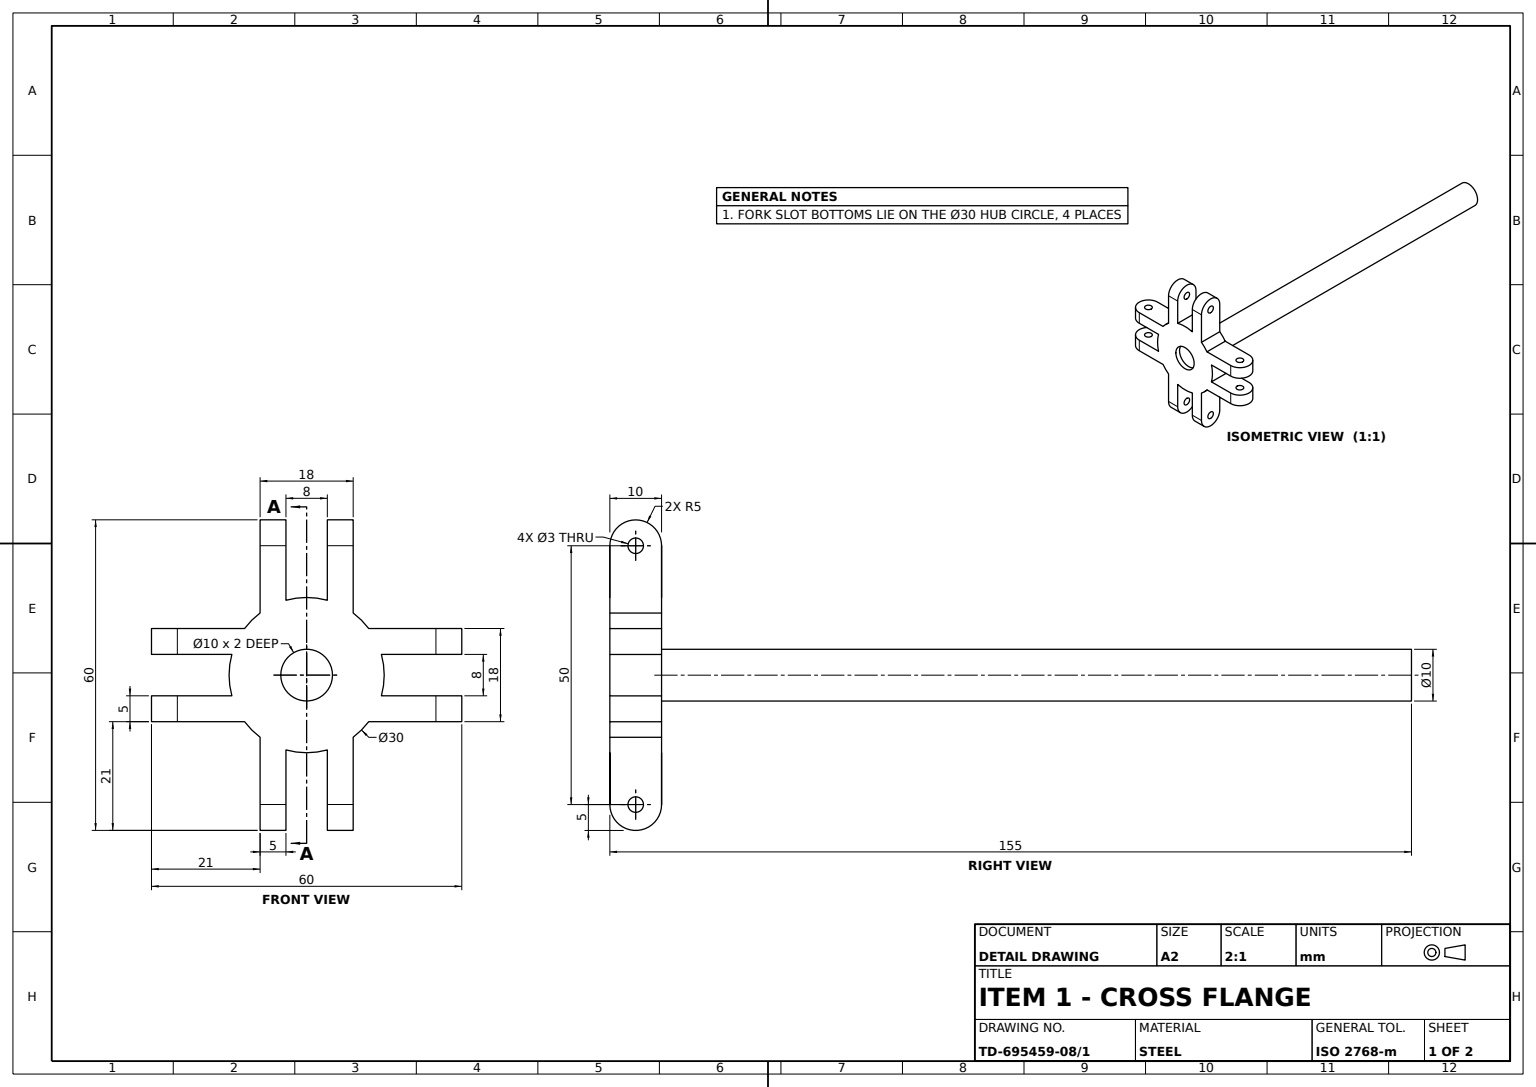
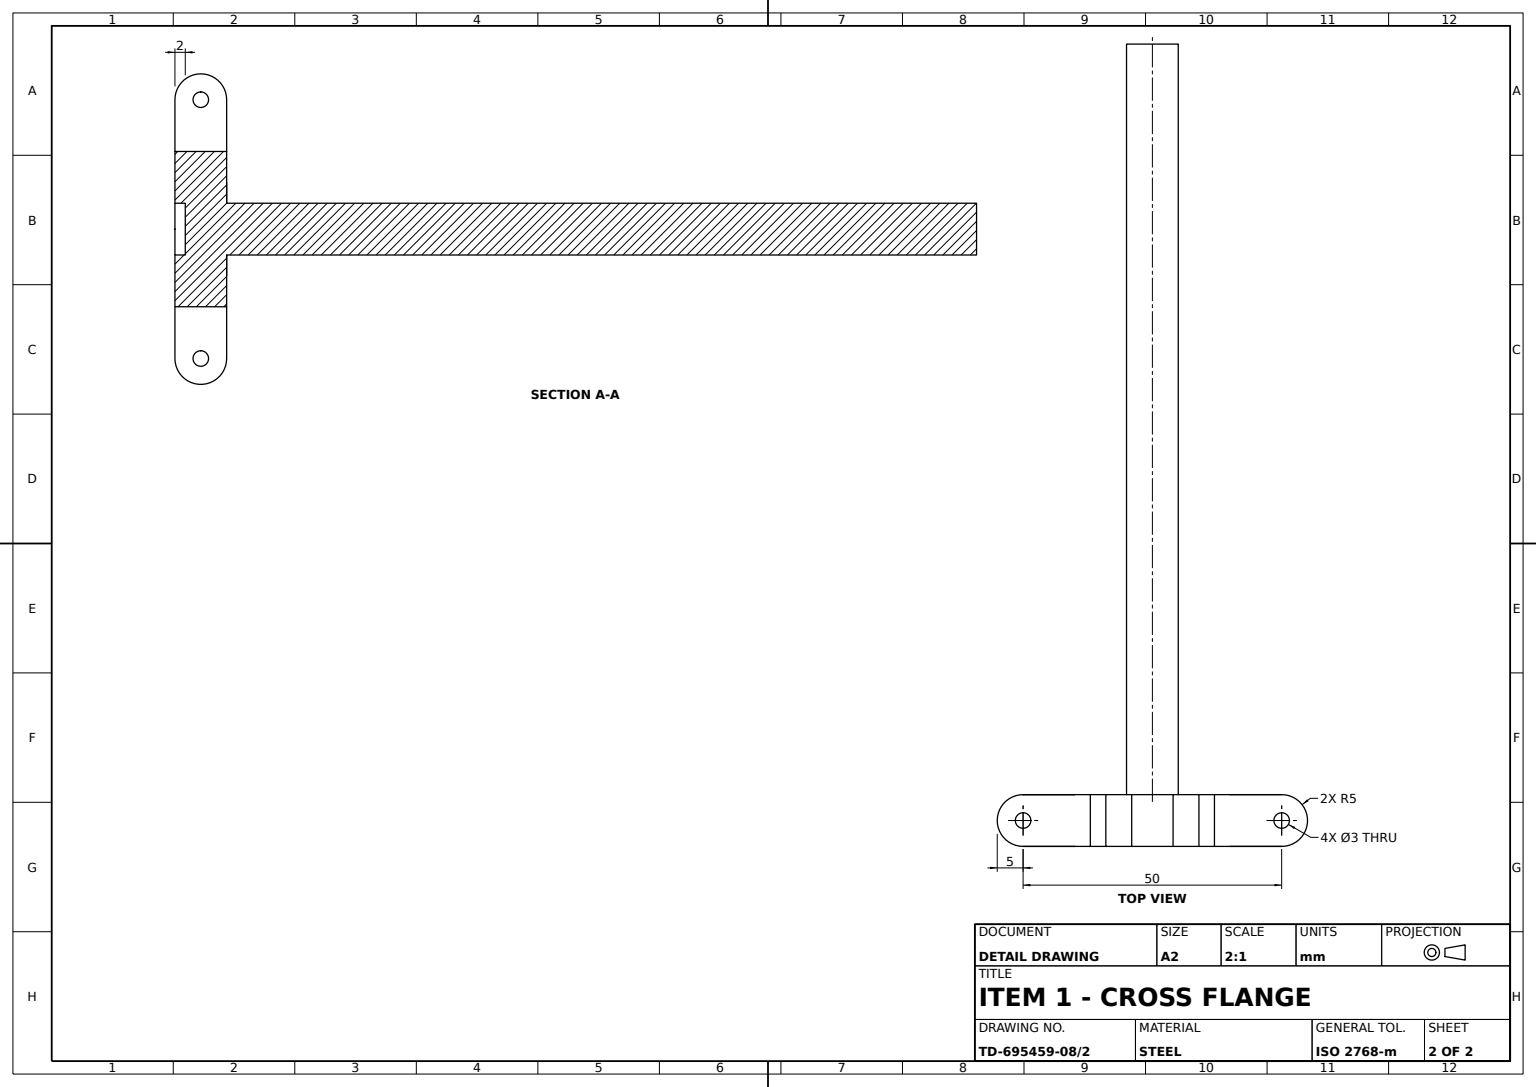
solid
v1 (-25,4,5)
v2 (-25,9,5)
e1 v1 v2 LINE
v3 (-30,9,0)
e2 v3 v2 CIRCLE(AX(P(-25,9,0),D(0,1,0),D(-1,0,0)),5)
v4 (-30,4,0)
e3 v4 v3 LINE
e4 v4 v1 CIRCLE(AX(P(-25,4,0),D(0,1,0),D(-1,0,0)),5)
face CYL(AX(P(-25,-30,0),D(0,1,0),D(-1,0,0)),5) [e1 -e2 -e3 e4]
v5 (25,-9,5)
v6 (25,-4,5)
e5 v5 v6 LINE
v7 (25,-9,-5)
e6 v7 v5 CIRCLE(AX(P(25,-9,0),D(0,-1,0),D(1,0,0)),5)
v8 (25,-4,-5)
e7 v7 v8 LINE
e8 v8 v6 CIRCLE(AX(P(25,-4,0),D(0,-1,0),D(1,0,0)),5)
face CYL(AX(P(25,-30,0),D(0,1,0),D(-1,0,0)),5) [-e5 -e6 e7 e8]
v9 (-26.5,9,0)
v10 (-23.5,9,0)
e9 v9 v10 CIRCLE(AX(P(-25,9,0),D(0,1,0),D(-1,0,0)),1.5)
v11 (-23.5,4,0)
e10 v11 v10 LINE
v12 (-26.5,4,0)
e11 v12 v11 CIRCLE(AX(P(-25,4,0),D(0,1,0),D(-1,0,0)),1.5)
e12 v12 v9 LINE
face CYL(AX(P(-25,-30,0),D(0,1,0),D(-1,0,0)),1.5) rev [e9 -e10 -e11 e12]
v13 (-12,9,5)
v14 (-12,9,-5)
e13 v13 v14 LINE
v15 (-9,12,5)
e14 v15 v13 CIRCLE(AX(P(0,0,5),D(0,0,1),D(1,0,0)),15)
v16 (-9,12,-5)
e15 v15 v16 LINE
e16 v16 v14 CIRCLE(AX(P(0,0,-5),D(0,0,1),D(1,0,0)),15)
face CYL(AX(P(0,0,5),D(0,0,-1),D(-1,0,0)),15) [-e13 -e14 e15 e16]
v17 (9,-25,5)
v18 (9,-12,5)
e17 v17 v18 LINE
v19 (9,-25,-5)
e18 v17 v19 CIRCLE(AX(P(9,-25,0),D(1,0,0),D(0,1,0)),5)
v20 (9,-12,-5)
e19 v19 v20 LINE
e20 v18 v20 LINE
v21 (9,-26.5,0)
v22 (9,-23.5,0)
e21 v21 v22 CIRCLE(AX(P(9,-25,0),D(1,0,0),D(0,1,0)),1.5)
e22 v22 v21 CIRCLE(AX(P(9,-25,0),D(1,0,0),D(0,1,0)),1.5)
face PLANE(AX(P(9,0,5),D(-1,0,0),D(0,-1,0))) rev [-e17 e18 e19 -e20] [-e21 -e22]
v23 (-5,0,5)
v24 (5,0,5)
e23 v23 v24 CIRCLE(AX(P(0,0,5),D(0,0,1),D(1,0,0)),5)
v25 (5,0,3)
e24 v25 v24 LINE
v26 (-5,0,3)
e25 v26 v25 CIRCLE(AX(P(0,0,3),D(0,0,1),D(1,0,0)),5)
e26 v26 v23 LINE
face CYL(AX(P(0,0,3),D(0,0,1),D(1,0,0)),5) rev [e23 -e24 -e25 e26]
v27 (12,-9,5)
v28 (12,-9,-5)
e27 v27 v28 LINE
e28 v7 v28 LINE
e29 v5 v27 LINE
v29 (23.5,-9,0)
v30 (26.5,-9,0)
e30 v29 v30 CIRCLE(AX(P(25,-9,0),D(0,-1,0),D(1,0,0)),1.5)
e31 v30 v29 CIRCLE(AX(P(25,-9,0),D(0,-1,0),D(1,0,0)),1.5)
face PLANE(AX(P(0,-9,5),D(0,-1,0),D(1,0,0))) [e27 -e28 e6 e29] [-e30 -e31]
v31 (-25,-4,-5)
v32 (-30,-4,0)
e32 v31 v32 CIRCLE(AX(P(-25,-4,0),D(0,1,0),D(-1,0,0)),5)
v33 (-25,-9,-5)
e33 v33 v31 LINE
v34 (-30,-9,0)
e34 v33 v34 CIRCLE(AX(P(-25,-9,0),D(0,1,0),D(-1,0,0)),5)
e35 v34 v32 LINE
face CYL(AX(P(-25,-30,0),D(0,1,0),D(-1,0,0)),5) [-e32 -e33 e34 e35]
v35 (-4,-25,-5)
v36 (-4,-14.456832,-5)
e36 v35 v36 LINE
v37 (-4,-14.456832,5)
e37 v37 v36 LINE
v38 (-4,-25,5)
e38 v38 v37 LINE
e39 v35 v38 CIRCLE(AX(P(-4,-25,0),D(-1,0,0),D(0,-1,0)),5)
v39 (-4,-23.5,0)
v40 (-4,-26.5,0)
e40 v39 v40 CIRCLE(AX(P(-4,-25,0),D(-1,0,0),D(0,-1,0)),1.5)
e41 v40 v39 CIRCLE(AX(P(-4,-25,0),D(-1,0,0),D(0,-1,0)),1.5)
face PLANE(AX(P(-4,0,5),D(-1,0,0),D(0,-1,0))) rev [e36 -e37 -e38 -e39] [e40 e41]
v41 (-4,26.5,0)
v42 (-4,23.5,0)
e42 v41 v42 CIRCLE(AX(P(-4,25,0),D(1,0,0),D(0,1,0)),1.5)
e43 v42 v41 CIRCLE(AX(P(-4,25,0),D(1,0,0),D(0,1,0)),1.5)
v43 (-4,25,-5)
v44 (-4,14.456832,-5)
e44 v43 v44 LINE
v45 (-4,30,0)
e45 v43 v45 CIRCLE(AX(P(-4,25,0),D(1,0,0),D(0,1,0)),5)
v46 (-4,25,5)
e46 v45 v46 CIRCLE(AX(P(-4,25,0),D(1,0,0),D(0,1,0)),5)
v47 (-4,14.456832,5)
e47 v46 v47 LINE
e48 v47 v44 LINE
face PLANE(AX(P(-4,0,5),D(1,0,0),D(0,1,0))) [-e42 -e43] [-e44 e45 e46 e47 e48]
v48 (25,9,-5)
v49 (12,9,-5)
e49 v48 v49 LINE
v50 (12,9,5)
e50 v50 v49 LINE
v51 (25,9,5)
e51 v51 v50 LINE
e52 v51 v48 CIRCLE(AX(P(25,9,0),D(0,1,0),D(-1,0,0)),5)
v52 (26.5,9,0)
v53 (23.5,9,0)
e53 v52 v53 CIRCLE(AX(P(25,9,0),D(0,1,0),D(-1,0,0)),1.5)
e54 v53 v52 CIRCLE(AX(P(25,9,0),D(0,1,0),D(-1,0,0)),1.5)
face PLANE(AX(P(0,9,5),D(0,-1,0),D(1,0,0))) rev [e49 -e50 -e51 e52] [-e53 -e54]
v54 (25,4,-5)
e55 v54 v48 LINE
v55 (14.456832,4,-5)
e56 v54 v55 LINE
v56 (14.456832,-4,-5)
e57 v56 v55 CIRCLE(AX(P(0,0,-5),D(0,0,1),D(1,0,0)),15)
e58 v8 v56 LINE
e59 v20 v28 CIRCLE(AX(P(0,0,-5),D(0,0,1),D(1,0,0)),15)
v57 (4,-25,-5)
e60 v57 v19 LINE
v58 (4,-14.456832,-5)
e61 v57 v58 LINE
e62 v36 v58 CIRCLE(AX(P(0,0,-5),D(0,0,1),D(1,0,0)),15)
v59 (-9,-25,-5)
e63 v59 v35 LINE
v60 (-9,-12,-5)
e64 v59 v60 LINE
v61 (-12,-9,-5)
e65 v61 v60 CIRCLE(AX(P(0,0,-5),D(0,0,1),D(1,0,0)),15)
e66 v33 v61 LINE
v62 (-14.456832,-4,-5)
e67 v31 v62 LINE
v63 (-15,0,-5)
e68 v63 v62 CIRCLE(AX(P(0,0,-5),D(0,0,1),D(1,0,0)),15)
v64 (-14.456832,4,-5)
e69 v64 v63 CIRCLE(AX(P(0,0,-5),D(0,0,1),D(1,0,0)),15)
v65 (-25,4,-5)
e70 v65 v64 LINE
v66 (-25,9,-5)
e71 v65 v66 LINE
e72 v66 v14 LINE
v67 (-9,25,-5)
e73 v67 v16 LINE
e74 v67 v43 LINE
v68 (4,14.456832,-5)
e75 v68 v44 CIRCLE(AX(P(0,0,-5),D(0,0,1),D(1,0,0)),15)
v69 (4,25,-5)
e76 v69 v68 LINE
v70 (9,25,-5)
e77 v69 v70 LINE
v71 (9,12,-5)
e78 v70 v71 LINE
e79 v49 v71 CIRCLE(AX(P(0,0,-5),D(0,0,1),D(1,0,0)),15)
v72 (5,0,-5)
v73 (-5,0,-5)
e80 v72 v73 CIRCLE(AX(P(0,0,-5),D(0,0,1),D(1,0,0)),5)
e81 v73 v72 CIRCLE(AX(P(0,0,-5),D(0,0,1),D(1,0,0)),5)
face PLANE(AX(P(0,0,-5),D(0,0,1),D(1,0,0))) rev [-e55 e56 -e57 -e58 -e7 e28 -e59 -e19 -e60 e61 -e62 -e36 -e63 e64 -e65 -e66 e33 e67 -e68 -e69 -e70 e71 e72 -e16 -e73 e74 e44 -e75 -e76 e77 e78 -e79 -e49] [e80 e81]
v74 (26.5,4,0)
v75 (23.5,4,0)
e82 v74 v75 CIRCLE(AX(P(25,4,0),D(0,-1,0),D(1,0,0)),1.5)
e83 v75 v53 LINE
e84 v74 v52 LINE
face CYL(AX(P(25,-30,0),D(0,1,0),D(-1,0,0)),1.5) rev [e82 e83 e54 -e84]
v76 (25,4,5)
e85 v76 v51 LINE
e86 v54 v76 CIRCLE(AX(P(25,4,0),D(0,-1,0),D(1,0,0)),5)
face CYL(AX(P(25,-30,0),D(0,1,0),D(-1,0,0)),5) [e55 -e52 -e85 -e86]
v77 (4,30,0)
e87 v69 v77 CIRCLE(AX(P(4,25,0),D(1,0,0),D(0,1,0)),5)
v78 (9,30,0)
e88 v77 v78 LINE
e89 v70 v78 CIRCLE(AX(P(9,25,0),D(1,0,0),D(0,1,0)),5)
face CYL(AX(P(-30,25,0),D(1,0,0),D(0,1,0)),5) [e87 e88 -e89 -e77]
e90 v25 v26 CIRCLE(AX(P(0,0,3),D(0,0,1),D(1,0,0)),5)
face PLANE(AX(P(0,0,3),D(0,0,1),D(1,0,0))) [e25 e90]
v79 (-5,0,-150)
v80 (5,0,-150)
e91 v79 v80 CIRCLE(AX(P(0,0,-150),D(0,0,1),D(1,0,0)),5)
e92 v80 v72 LINE
e93 v79 v73 LINE
face CYL(AX(P(0,0,-150),D(0,0,1),D(1,0,0)),5) [e91 e92 -e81 -e93]
e94 v75 v74 CIRCLE(AX(P(25,4,0),D(0,-1,0),D(1,0,0)),1.5)
v81 (14.456832,4,5)
e95 v76 v81 LINE
e96 v81 v55 LINE
face PLANE(AX(P(0,4,5),D(0,-1,0),D(1,0,0))) [-e82 -e94] [-e56 e86 e95 e96]
v82 (-15,0,5)
e97 v82 v63 LINE
v83 (-14.456832,-4,5)
e98 v83 v62 LINE
e99 v82 v83 CIRCLE(AX(P(0,0,5),D(0,0,1),D(1,0,0)),15)
face CYL(AX(P(0,0,5),D(0,0,-1),D(-1,0,0)),15) [e97 e68 -e98 -e99]
v84 (-14.456832,4,5)
e100 v84 v64 LINE
e101 v1 v84 LINE
e102 v65 v4 CIRCLE(AX(P(-25,4,0),D(0,1,0),D(-1,0,0)),5)
e103 v11 v12 CIRCLE(AX(P(-25,4,0),D(0,1,0),D(-1,0,0)),1.5)
face PLANE(AX(P(0,4,5),D(0,1,0),D(-1,0,0))) rev [-e100 -e101 -e4 -e102 e70] [e11 e103]
v85 (4,14.456832,5)
e104 v85 v68 LINE
v86 (4,25,5)
e105 v86 v85 LINE
e106 v77 v86 CIRCLE(AX(P(4,25,0),D(1,0,0),D(0,1,0)),5)
v87 (4,26.5,0)
v88 (4,23.5,0)
e107 v87 v88 CIRCLE(AX(P(4,25,0),D(1,0,0),D(0,1,0)),1.5)
e108 v88 v87 CIRCLE(AX(P(4,25,0),D(1,0,0),D(0,1,0)),1.5)
face PLANE(AX(P(4,0,5),D(1,0,0),D(0,1,0))) rev [-e87 e76 -e104 -e105 -e106] [e107 e108]
e109 v66 v3 CIRCLE(AX(P(-25,9,0),D(0,1,0),D(-1,0,0)),5)
face CYL(AX(P(-25,-30,0),D(0,1,0),D(-1,0,0)),5) [-e71 e102 e3 -e109]
v89 (4,-26.5,0)
e110 v89 v21 LINE
v90 (4,-23.5,0)
e111 v90 v22 LINE
e112 v90 v89 CIRCLE(AX(P(4,-25,0),D(-1,0,0),D(0,-1,0)),1.5)
face CYL(AX(P(-30,-25,0),D(1,0,0),D(0,1,0)),1.5) rev [e110 e21 -e111 e112]
e113 v84 v82 CIRCLE(AX(P(0,0,5),D(0,0,1),D(1,0,0)),15)
face CYL(AX(P(0,0,5),D(0,0,-1),D(-1,0,0)),15) [e100 e69 -e97 -e113]
v91 (-9,-25,5)
e114 v91 v38 LINE
e115 v59 v91 CIRCLE(AX(P(-9,-25,0),D(-1,0,0),D(0,-1,0)),5)
face CYL(AX(P(-30,-25,0),D(1,0,0),D(0,1,0)),5) [-e114 -e115 e63 e39]
v92 (-9,30,0)
e116 v92 v45 LINE
e117 v67 v92 CIRCLE(AX(P(-9,25,0),D(1,0,0),D(0,1,0)),5)
face CYL(AX(P(-30,25,0),D(1,0,0),D(0,1,0)),5) [e116 -e45 -e74 e117]
v93 (9,12,5)
e118 v93 v71 LINE
e119 v50 v93 CIRCLE(AX(P(0,0,5),D(0,0,1),D(1,0,0)),15)
face CYL(AX(P(0,0,5),D(0,0,-1),D(-1,0,0)),15) [e79 -e118 -e119 e50]
e120 v80 v79 CIRCLE(AX(P(0,0,-150),D(0,0,1),D(1,0,0)),5)
face CYL(AX(P(0,0,-150),D(0,0,1),D(1,0,0)),5) [e120 e93 -e80 -e92]
v94 (9,25,5)
e121 v78 v94 CIRCLE(AX(P(9,25,0),D(1,0,0),D(0,1,0)),5)
e122 v94 v93 LINE
v95 (9,23.5,0)
v96 (9,26.5,0)
e123 v95 v96 CIRCLE(AX(P(9,25,0),D(1,0,0),D(0,1,0)),1.5)
e124 v96 v95 CIRCLE(AX(P(9,25,0),D(1,0,0),D(0,1,0)),1.5)
face PLANE(AX(P(9,0,5),D(1,0,0),D(0,1,0))) [-e78 e89 e121 e122 e118] [-e123 -e124]
v97 (-9,25,5)
e125 v92 v97 CIRCLE(AX(P(-9,25,0),D(1,0,0),D(0,1,0)),5)
e126 v97 v46 LINE
face CYL(AX(P(-30,25,0),D(1,0,0),D(0,1,0)),5) [e125 e126 -e46 -e116]
v98 (14.456832,-4,5)
e127 v98 v81 CIRCLE(AX(P(0,0,5),D(0,0,1),D(1,0,0)),15)
e128 v98 v56 LINE
face CYL(AX(P(0,0,5),D(0,0,-1),D(-1,0,0)),15) [-e127 e128 e57 -e96]
v99 (23.5,-4,0)
e129 v29 v99 LINE
v100 (26.5,-4,0)
e130 v100 v99 CIRCLE(AX(P(25,-4,0),D(0,-1,0),D(1,0,0)),1.5)
e131 v30 v100 LINE
face CYL(AX(P(25,-30,0),D(0,1,0),D(-1,0,0)),1.5) rev [e31 e129 -e130 -e131]
v101 (-25,-4,5)
e132 v32 v101 CIRCLE(AX(P(-25,-4,0),D(0,1,0),D(-1,0,0)),5)
e133 v101 v83 LINE
v102 (-26.5,-4,0)
v103 (-23.5,-4,0)
e134 v102 v103 CIRCLE(AX(P(-25,-4,0),D(0,1,0),D(-1,0,0)),1.5)
e135 v103 v102 CIRCLE(AX(P(-25,-4,0),D(0,1,0),D(-1,0,0)),1.5)
face PLANE(AX(P(0,-4,5),D(0,1,0),D(-1,0,0))) [e32 e132 e133 e98 -e67] [-e134 -e135]
v104 (-9,-12,5)
e136 v91 v104 LINE
e137 v104 v60 LINE
v105 (-9,-26.5,0)
v106 (-9,-23.5,0)
e138 v105 v106 CIRCLE(AX(P(-9,-25,0),D(-1,0,0),D(0,-1,0)),1.5)
e139 v106 v105 CIRCLE(AX(P(-9,-25,0),D(-1,0,0),D(0,-1,0)),1.5)
face PLANE(AX(P(-9,0,5),D(-1,0,0),D(0,-1,0))) [e136 e137 -e64 e115] [-e138 -e139]
v107 (4,-25,5)
e140 v107 v17 LINE
e141 v57 v107 CIRCLE(AX(P(4,-25,0),D(-1,0,0),D(0,-1,0)),5)
face CYL(AX(P(-30,-25,0),D(1,0,0),D(0,1,0)),5) [-e140 -e141 e60 -e18]
e142 v106 v39 LINE
e143 v105 v40 LINE
face CYL(AX(P(-30,-25,0),D(1,0,0),D(0,1,0)),1.5) rev [-e40 -e142 e139 e143]
v108 (-23.5,-9,0)
v109 (-26.5,-9,0)
e144 v108 v109 CIRCLE(AX(P(-25,-9,0),D(0,1,0),D(-1,0,0)),1.5)
e145 v108 v103 LINE
e146 v109 v102 LINE
face CYL(AX(P(-25,-30,0),D(0,1,0),D(-1,0,0)),1.5) rev [-e144 e145 e135 -e146]
e147 v109 v108 CIRCLE(AX(P(-25,-9,0),D(0,1,0),D(-1,0,0)),1.5)
v110 (-12,-9,5)
e148 v110 v61 LINE
v111 (-25,-9,5)
e149 v111 v110 LINE
e150 v34 v111 CIRCLE(AX(P(-25,-9,0),D(0,1,0),D(-1,0,0)),5)
face PLANE(AX(P(0,-9,5),D(0,1,0),D(-1,0,0))) rev [e144 e147] [-e148 -e149 -e150 -e34 e66]
e151 v111 v101 LINE
e152 v110 v104 CIRCLE(AX(P(0,0,5),D(0,0,1),D(1,0,0)),15)
v112 (4,-14.456832,5)
e153 v37 v112 CIRCLE(AX(P(0,0,5),D(0,0,1),D(1,0,0)),15)
e154 v107 v112 LINE
e155 v18 v27 CIRCLE(AX(P(0,0,5),D(0,0,1),D(1,0,0)),15)
e156 v6 v98 LINE
e157 v86 v94 LINE
e158 v85 v47 CIRCLE(AX(P(0,0,5),D(0,0,1),D(1,0,0)),15)
e159 v97 v15 LINE
e160 v2 v13 LINE
e161 v24 v23 CIRCLE(AX(P(0,0,5),D(0,0,1),D(1,0,0)),5)
face PLANE(AX(P(0,0,5),D(0,0,1),D(1,0,0))) [e101 e113 e99 -e133 -e151 e149 e152 -e136 e114 e38 e153 -e154 e140 e17 e155 -e29 e5 e156 e127 -e95 e85 e51 e119 -e122 -e157 e105 e158 -e47 -e126 e159 e14 -e160 -e1] [-e161 -e23]
face CYL(AX(P(0,0,5),D(0,0,-1),D(-1,0,0)),15) [e104 e75 -e48 -e158]
e162 v99 v100 CIRCLE(AX(P(25,-4,0),D(0,-1,0),D(1,0,0)),1.5)
face PLANE(AX(P(0,-4,5),D(0,-1,0),D(1,0,0))) rev [e130 e162] [-e8 e58 -e128 -e156]
e163 v10 v9 CIRCLE(AX(P(-25,9,0),D(0,1,0),D(-1,0,0)),1.5)
face CYL(AX(P(-25,-30,0),D(0,1,0),D(-1,0,0)),1.5) rev [e10 e163 -e12 -e103]
e164 v89 v90 CIRCLE(AX(P(4,-25,0),D(-1,0,0),D(0,-1,0)),1.5)
e165 v112 v58 LINE
face PLANE(AX(P(4,0,5),D(-1,0,0),D(0,-1,0))) [-e164 -e112] [-e61 e141 e154 e165]
face CYL(AX(P(-25,-30,0),D(0,1,0),D(-1,0,0)),5) [e150 e151 -e132 -e35]
v113 (-9,26.5,0)
e166 v113 v41 LINE
v114 (-9,23.5,0)
e167 v114 v113 CIRCLE(AX(P(-9,25,0),D(1,0,0),D(0,1,0)),1.5)
e168 v114 v42 LINE
face CYL(AX(P(-30,25,0),D(1,0,0),D(0,1,0)),1.5) rev [e43 -e166 -e167 e168]
face CYL(AX(P(0,0,5),D(0,0,-1),D(-1,0,0)),15) [e59 -e27 -e155 e20]
face CYL(AX(P(-30,-25,0),D(1,0,0),D(0,1,0)),1.5) rev [e164 e111 e22 -e110]
face CYL(AX(P(25,-30,0),D(0,1,0),D(-1,0,0)),1.5) rev [e131 -e162 -e129 e30]
e169 v113 v114 CIRCLE(AX(P(-9,25,0),D(1,0,0),D(0,1,0)),1.5)
face PLANE(AX(P(-9,0,5),D(1,0,0),D(0,1,0))) rev [-e125 -e117 e73 -e15 -e159] [e167 e169]
face CYL(AX(P(-30,25,0),D(1,0,0),D(0,1,0)),1.5) rev [-e169 e166 e42 -e168]
e170 v87 v96 LINE
e171 v88 v95 LINE
face CYL(AX(P(-30,25,0),D(1,0,0),D(0,1,0)),1.5) rev [-e170 -e108 e171 e123]
face CYL(AX(P(-30,25,0),D(1,0,0),D(0,1,0)),5) [e157 -e121 -e88 e106]
face CYL(AX(P(-25,-30,0),D(0,1,0),D(-1,0,0)),1.5) rev [e146 e134 -e145 -e147]
face CYL(AX(P(0,0,5),D(0,0,-1),D(-1,0,0)),15) [e62 -e165 -e153 e37]
face PLANE(AX(P(0,0,-150),D(0,0,1),D(1,0,0))) rev [-e120 -e91]
face CYL(AX(P(0,0,3),D(0,0,1),D(1,0,0)),5) rev [e24 e161 -e26 -e90]
face CYL(AX(P(25,-30,0),D(0,1,0),D(-1,0,0)),1.5) rev [e84 e53 -e83 e94]
face CYL(AX(P(-30,-25,0),D(1,0,0),D(0,1,0)),1.5) rev [e142 -e41 -e143 e138]
face PLANE(AX(P(0,9,5),D(0,1,0),D(-1,0,0))) [e109 e2 e160 e13 -e72] [-e163 -e9]
face CYL(AX(P(-30,25,0),D(1,0,0),D(0,1,0)),1.5) rev [-e107 e170 e124 -e171]
face CYL(AX(P(0,0,5),D(0,0,-1),D(-1,0,0)),15) [e148 e65 -e137 -e152]
